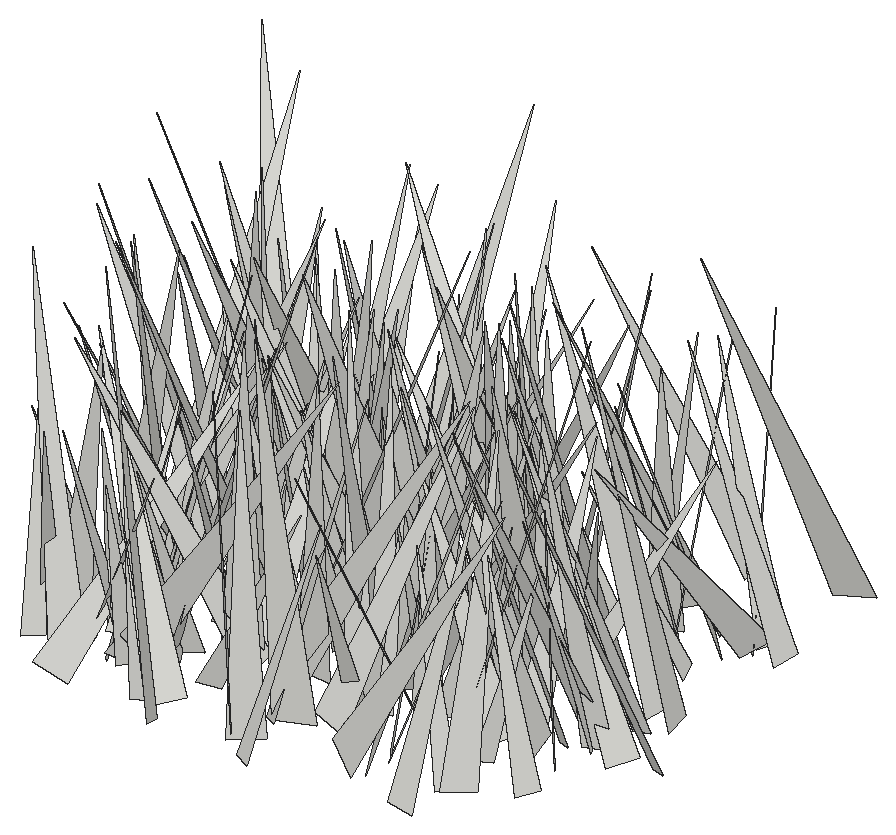
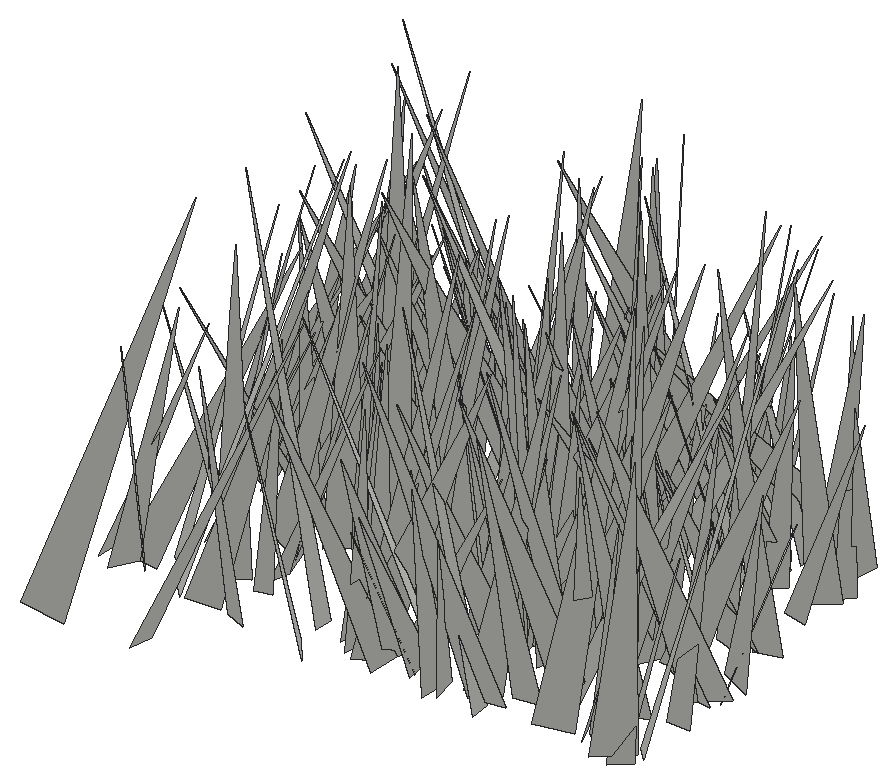
# SketchUp Ruby script. Lengths in inches.
U = 1.inch
M = Sketchup.active_model
def pt(a) = Geom::Point3d.new(a.map { |v| v * U })
def face(e, loops, mat)
  f = e.add_face(loops[0].map { |a| pt(a) })
  loops[1..].each { |l| e.add_face(l.map { |a| pt(a) }).erase! }
  f.material = f.back_material = mat if mat
  f
end
# faces: each face lists its corners as indices into pts; further lists are holes
def faces(e, pts, list, mat = nil) = list.each { |f| face(e, (f[0].is_a?(Array) ? f : [f]).map { |l| l.map { |i| pts[i] } }, mat) }
# xy, xz, yz: faces in a plane at the given z, y or x. An outline is a flat list of corners, or four numbers for a rectangle; further outlines are holes
def ring(l) = l.size == 4 ? [[l[0], l[1]], [l[2], l[1]], [l[2], l[3]], [l[0], l[3]]] : l.each_slice(2).to_a
def flat(e, list, mat, &to3) = list.each { |f| face(e, (f[0].is_a?(Array) ? f : [f]).map { |l| ring(l).map { |u, v| to3.(u, v) } }, mat) }
def xy(e, z, list, mat = nil) = flat(e, list, mat) { |x, y| [x, y, z] }
def xz(e, y, list, mat = nil) = flat(e, list, mat) { |x, z| [x, y, z] }
def yz(e, x, list, mat = nil) = flat(e, list, mat) { |y, z| [x, y, z] }
def lines(e, pts, list) = list.each { |a, b| e.add_line(pt(pts[a]), pt(pts[b])) }
# prism: a flat outline (further loops are holes) pulled along v
def prism(e, loops, v, mat = nil)
  f = face(e, loops, mat); d = Geom::Vector3d.new(v.map { |x| x * U })
  f.pushpull(f.normal.samedirection?(d) ? d.length : -d.length)
end
def box(e, o, s, mat = nil) = prism(e, [[o, [o[0] + s[0], o[1], o[2]], [o[0] + s[0], o[1] + s[1], o[2]], [o[0], o[1] + s[1], o[2]]]], [0, 0, s[2]], mat)
def at(x, y, z, deg = 0) = Geom::Transformation.translation(pt([x, y, z])) * Geom::Transformation.rotation(ORIGIN, Z_AXIS, deg.degrees)
def axes(o, x, y, z) = Geom::Transformation.new([*x, 0, *y, 0, *z, 0, *pt(o).to_a, 1])
def part(name) = M.definitions.add(name)
# library, detail: a bought-in or finely detailed component or shape, given as its bounding box
def library(name, o, s) = part(name).tap { |d| box(d.entities, o, s) }
def detail(e, o, s) = box(e.add_group.entities, o, s)
def put(e, d, t, mat = nil) = e.add_instance(d, t).tap { |i| i.material = mat if mat }
def group(e, t, mat = nil) = e.add_group.tap { |g| g.transformation = t; g.material = mat if mat }.entities
root = M.entities
c1 = part("fur_instance\#9")
p = [[0.8125,0,1.79],[0.67,-0.02,1.48],[0,-0.11,0],[0,0.11,0]]
faces(c1.entities,p,[[0,1,2,3]])
put(root,c1,axes([75.72,306.375,-27.1],[4.83002,3.67653,3.08875],[4.26917,-5.29337,-0.3752],[-2.19806,-2.20219,6.05848]))
put(root,c1,axes([76.89,305.76,-27.1],[3.45962,-4.50001,2.91683],[-5.02174,-3.93643,-0.1168],[-1.88153,2.2319,5.67498]))
put(root,c1,axes([77.69,304.53,-27.1],[2.30646,3.84948,0.31393],[3.83736,-2.32546,0.32205],[-0.43787,-0.10267,4.47599]))
put(root,c1,axes([80.25,306.78,-27.1],[3.77376,6.10396,1.49671],[5.76595,-2.66802,-3.65722],[2.50047,-3.05991,6.17449]))
put(root,c1,axes([72.33,305.65,-27.1],[-0.0394,4.36961,1.02441],[4.32756,-0.23455,1.1669],[-1.18959,-0.99797,4.2111]))
put(root,c1,axes([70.46,307.35,-27.1],[2.53184,-2.74895,1.13947],[-2.76231,-2.72751,-0.44237],[-1.1067,0.51894,3.71097]))
put(root,c1,axes([69.88,308.06,-27.1],[-4.44345,-1.97155,1.25823],[-1.71315,4.58269,1.13072],[1.59225,-0.57131,4.72787]))
put(root,c1,axes([73.58,304.73,-27.1],[-7.24108,-2.76695,1.69952],[-3.23599,6.49389,-3.21487],[0.2698,3.62643,7.05364]))
put(root,c1,axes([83.98,305.26,-27.1],[1.01663,5.56132,0.68679],[5.60282,-1.02017,-0.03274],[-0.09106,-0.68151,5.65338]))
put(root,c1,axes([68.67,307.44,-27.1],[4.5818,0.64032,0.1617],[0.65902,-4.5067,-0.82732],[-0.04299,-0.84188,4.55176]))
put(root,c1,axes([66.07,308.64,-27.1],[4.73789,-1.18845,0.72275],[-0.9672,-4.65874,-1.32025],[-0.99966,-1.12521,4.70287]))
put(root,c1,axes([77.43,307.71,-27.1],[-2.10134,6.53759,3.4605],[7.38552,2.05442,0.60354],[0.41142,-3.48856,6.84043]))
put(root,c1,axes([81.06,307.31,-27.1],[7.00496,3.81978,0.96353],[3.93839,-6.83549,-1.53416],[-0.09034,-1.80938,7.82984]))
put(root,c1,axes([73.15,306.09,-27.1],[-5.62336,3.63446,0.06059],[3.63174,5.6129,0.37548],[-0.15301,-0.3482,6.6851]))
put(root,c1,axes([78.87,309.48,-27.1],[0.77798,-4.23548,0.16889],[-4.23878,-0.77834,0.00619],[-0.02442,0.16723,4.30633]))
put(root,c1,axes([84.37,307.36,-27.1],[-3.97928,1.73175,0.54979],[1.73454,4.01483,-0.09183],[0.54094,-0.13447,4.3388]))
put(root,c1,axes([73.53,307.9,-27.1],[3.09859,-2.8989,0.71648],[-2.92503,-2.73871,1.56906],[0.60101,1.61681,3.94246]))
put(root,c1,axes([70.34,307.41,-27.1],[5.69226,-5.26322,0.96159],[-5.00885,-4.7486,3.65927],[1.88086,3.28288,6.8347]))
put(root,c1,axes([71.4,309.11,-27.1],[-5.49942,-3.45806,0.94275],[-3.51329,5.5426,-0.16378],[0.70973,0.64178,6.49422]))
put(root,c1,axes([74.0625,309.9375,-27.1],[-7.08449,-0.21202,0.14595],[-0.16992,6.87165,1.73429],[0.19334,-1.72965,6.8722]))
put(root,c1,axes([66.67,306.9,-27.1],[-4.24883,1.88722,0.42776],[1.75815,4.19597,-1.04876],[0.80838,0.79335,4.52927]))
put(root,c1,axes([80.23,310.84,-27.1],[-3.47678,-4.99975,0.07246],[-4.93171,3.44331,0.95532],[0.82523,-0.48669,6.01439]))
put(root,c1,axes([79.46,308.47,-27.1],[1.72384,-3.5656,0.8716],[-3.29525,-1.07913,2.10276],[1.61693,1.60212,3.35612]))
put(root,c1,axes([71.69,309.38,-27.1],[0.72019,-3.80208,0.86926],[-3.795,-0.88705,-0.73566],[-0.89965,0.69817,3.79912]))
put(root,c1,axes([68.43,309.53,-27.1],[3.6116,-2.54944,1.03868],[-2.46348,-3.75778,-0.65768],[-1.22872,0.0404,4.37159]))
put(root,c1,axes([68.17,306.91,-27.1],[-6.64184,2.29308,0.28161],[2.23011,6.58737,-1.04152],[0.60342,0.8944,6.94892]))
put(root,c1,axes([66.43,309.35,-27.1],[2.75053,-5.09352,1.52718],[-5.31748,-2.64324,0.76119],[-0.02665,1.70616,5.73847]))
put(root,c1,axes([86.78,308.78,-27.1],[-3.90024,1.94852,0.94584],[2.05782,3.9414,0.36592],[0.67579,-0.75618,4.3445]))
put(root,c1,axes([68.76,305.23,-27.1],[-3.50989,5.55769,0.51718],[4.45011,3.15505,-3.70364],[3.36927,1.62248,5.4305]))
put(root,c1,axes([73.36,309.95,-27.1],[4.72126,-4.87179,1.88096],[-5.03873,-4.91595,-0.08523],[-1.37242,1.28908,6.78361]))
put(root,c1,axes([75.08,309.59,-27.1],[4.55418,4.59674,3.34406],[5.23121,-5.06575,-0.16086],[-2.22422,-2.50228,6.46875]))
put(root,c1,axes([84.8,307.46,-27.1],[-5.4201,3.31702,1.28358],[3.06796,5.54385,-1.37151],[1.7994,0.53923,6.20476]))
put(root,c1,axes([69.67,307.125,-27.1],[3.36886,3.17868,0.5186],[2.75759,-3.23451,1.91201],[-1.66392,1.0752,4.2187]))
put(root,c1,axes([85.1,311.53,-27.1],[-7.14717,-1.7401,1.8273],[-1.33254,7.26397,1.70532],[2.14274,-1.28679,7.15555]))
put(root,c1,axes([75.9,310.64,-27.1],[0.59547,-6.22896,1.95156],[-6.50827,-0.41619,0.65745],[0.50087,1.99748,6.22272]))
put(root,c1,axes([66.56,310.77,-27.1],[-0.08918,-3.86635,0.81214],[-3.84672,-0.10019,-0.89937],[-0.90053,0.81086,3.76135]))
put(root,c1,axes([76.6875,307.3,-27.1],[3.68113,4.53912,0.36663],[4.24955,-3.59341,1.82137],[-1.63686,0.87892,5.5531]))
put(root,c1,axes([78.4375,308.35,-27.1],[1.11802,6.55656,0.88639],[6.4324,-0.86675,-1.70208],[1.54866,-1.13332,6.42972]))
put(root,c1,axes([81.57,307.78,-27.1],[4.34106,2.99141,0.28027],[2.79242,-4.19877,1.56351],[-1.10882,1.13738,5.03476]))
put(root,c1,axes([75.03,310.71,-27.1],[4.40787,6.56573,1.54887],[6.23945,-3.26461,-3.91775],[2.5646,-3.34225,6.86945]))
put(root,c1,axes([71.49,312.16,-27.1],[-3.69679,-5.87263,0.02895],[-5.78236,3.6339,-1.23044],[-1.02613,0.67962,6.82936]))
put(root,c1,axes([84.16,309.57,-27.1],[3.26385,-1.40609,1.47007],[-1.85279,-3.20219,1.05074],[-0.83985,1.59994,3.39496]))
put(root,c1,axes([83.07,309.98,-27.1],[4.24313,0.45781,1.20359],[0.34307,-4.39664,0.46288],[-1.24117,0.34981,4.24258]))
put(root,c1,axes([81.36,308.08,-27.1],[4.43621,4.25023,1.48293],[3.65379,-4.61591,2.29927],[-2.62932,0.75659,5.69717]))
put(root,c1,axes([69.42,310.12,-27.1],[6.44327,3.68852,1.42181],[3.82977,-6.4983,-0.49739],[-0.97955,-1.14429,7.40767]))
put(root,c1,axes([76.3,308.55,-27.1],[-6.09623,-2.24198,1.5344],[-2.70516,5.35755,-2.91953],[0.25098,3.28863,5.80232]))
put(root,c1,axes([68.91,308.79,-27.1],[-2.94733,3.27814,0.42411],[3.06608,2.92358,-1.29021],[1.23501,0.56503,4.21525]))
put(root,c1,axes([79.3,310.16,-27.1],[-0.34348,3.88251,1.09091],[4.02925,0.37671,-0.07204],[0.17064,-1.07988,3.89701]))
put(root,c1,axes([74.78,311.33,-27.1],[2.18952,-4.24382,2.13551],[-4.35668,-2.73133,-0.96101],[-1.89466,1.3763,4.67766]))
put(root,c1,axes([86.23,313.35,-27.1],[-1.07248,-7.00957,0.36815],[-6.96342,1.01561,-0.94825],[-0.88342,0.50425,7.02746]))
put(root,c1,axes([70.2,313.06,-27.1],[-1.799,-4.93024,0.4482],[-4.7112,1.85147,1.45641],[1.52075,-0.09654,5.04207]))
put(root,c1,axes([73.57,312.09,-27.1],[-3.74944,-6.99723,1.04952],[-6.92154,3.38084,-2.18706],[-1.468,1.93125,7.63127]))
put(root,c1,axes([86.12,311.03,-27.1],[3.3067,2.95122,2.18217],[3.23124,-3.73382,0.15332],[-1.74087,-1.32466,4.4295]))
put(root,c1,axes([83.76,311.19,-27.1],[-3.5373,3.73043,1.14853],[3.88761,3.22863,1.48666],[-0.34887,-1.84596,4.92122]))
put(root,c1,axes([82.12,312.63,-27.1],[3.81403,-1.87609,0.65313],[-1.66249,-3.78837,-1.17367],[-1.0874,-0.78844,4.08523]))
put(root,c1,axes([71.63,308.04,-27.1],[6.96857,3.90701,1.2479],[3.36407,-6.85211,2.66731],[-2.34628,1.77954,7.53068]))
put(root,c1,axes([76.64,313.21,-27.1],[6.75782,0.35235,2.65885],[1.16075,-6.88187,-2.03823],[-2.41791,-2.31896,6.45275]))
put(root,c1,axes([80.28,311.41,-27.1],[3.33409,-2.8819,1.80128],[-3.12207,-3.59416,0.02846],[-1.34262,1.20116,4.40689]))
put(root,c1,axes([72.57,312.99,-27.1],[2.27929,-4.31761,0.37807],[-4.29346,-2.30768,-0.46977],[-0.59235,0.11282,4.85966]))
put(root,c1,axes([79.76,312.16,-27.1],[-0.47471,-3.8388,0.84095],[-3.92781,0.49062,0.02236],[0.12592,0.83177,3.86797]))
put(root,c1,axes([83.41,308.91,-27.1],[6.6915,4.26773,1.20587],[3.94044,-6.72308,1.92792],[-2.03484,1.01512,7.69888]))
put(root,c1,axes([86.33,312.93,-27.1],[-4.22717,-2.44585,1.01456],[-2.28976,4.33627,0.91336],[1.32985,-0.3083,4.79759]))
put(root,c1,axes([67.24,313.69,-27.1],[-3.46246,-6.72611,1.90114],[-6.59046,3.84836,1.61233],[2.32826,0.89059,7.39118]))
put(root,c1,axes([75.32,312.98,-27.1],[3.88583,-1.17381,1.38743],[-0.79486,-4.04284,-1.19419],[-1.63432,-0.82466,3.87962]))
put(root,c1,axes([72.09,312.71,-27.1],[1.922,-3.18961,0.22781],[-3.1707,-1.86642,0.61867],[0.41494,0.51232,3.67219]))
put(root,c1,axes([68.85,311.06,-27.1],[3.76051,3.97563,0.83952],[4.01253,-3.81366,0.08642],[-0.64034,-0.54974,5.47171]))
put(root,c1,axes([89.28,312.75,-27.1],[-4.75874,-5.64309,0.42264],[-5.39038,4.3522,-2.58279],[-1.72245,1.97043,6.91515]))
put(root,c1,axes([85.59,312.22,-27.1],[-3.98273,-4.40716,0.90523],[-4.3967,3.55588,-2.0321],[-0.95477,2.0093,5.58174]))
put(root,c1,axes([75.32,313.49,-27.1],[3.57581,-3.48366,1.446],[-3.33217,-3.85124,-1.03819],[-1.76733,0.21279,4.88308]))
put(root,c1,axes([86.68,312.71,-27.1],[0.19192,-5.71021,2.24229],[-6.02696,-0.59408,-0.99702],[-1.14462,2.17066,5.62577]))
put(root,c1,axes([71.11,311.5,-27.1],[3.02903,2.92229,1.12241],[2.89072,-3.2105,0.55771],[-1.2014,-0.35704,4.17178]))
put(root,c1,axes([76.66,312.27,-27.1],[4.45392,4.12687,0.87812],[4.21021,-4.26347,-1.31776],[0.27618,-1.55927,5.92722]))
put(root,c1,axes([81.53,313.84,-27.1],[2.47243,-7.62212,2.09201],[-7.90302,-2.41845,0.52868],[-0.12434,2.1542,7.99563]))
put(root,c1,axes([65.71,313.32,-27.1],[-0.42435,-6.57592,2.54627],[-6.78158,1.0798,1.65847],[1.93298,2.34469,6.37748]))
put(root,c1,axes([82.26,315.08,-27.1],[5.27875,-5.42072,0.96709],[-5.29735,-5.36505,-1.15714],[-1.50251,-0.12916,7.47733]))
put(root,c1,axes([77.51,311.14,-27.1],[0.02975,6.47261,1.15989],[6.34372,-0.33363,1.69906],[-1.73125,-1.11127,6.2457]))
put(root,c1,axes([78.87,309.45,-27.1],[7.42059,-0.17453,3.00871],[-1.57677,-7.03899,3.48057],[-2.56838,3.81708,6.55601]))
put(root,c1,axes([78.27,311.49,-27.1],[-5.05186,2.37101,0.85511],[2.22237,5.09377,-0.9944],[1.18912,0.55319,5.49128]))
put(root,c1,axes([73.49,313.56,-27.1],[-2.97615,-4.05495,1.48787],[-4.26463,3.04523,-0.23114],[0.68511,1.34083,5.02461]))
put(root,c1,axes([79.25,312.14,-27.1],[6.564,-1.73993,0.0582],[-1.67851,-6.26496,2.01239],[0.46191,1.95953,6.48565]))
put(root,c1,axes([68.47,313.28,-27.1],[4.49917,3.28934,0.87918],[3.40387,-4.3112,-1.28935],[0.07989,-1.55853,5.42216]))
put(root,c1,axes([84.3,311.85,-27.1],[-1.65909,5.33475,1.21269],[5.33342,1.85943,-0.88312],[1.21852,-0.87506,5.51654]))
put(root,c1,axes([70.81,315.15,-27.1],[-0.56005,-4.94681,0.27227],[-4.82604,0.60667,1.09544],[1.12,0.14049,4.85639]))
put(root,c1,axes([71.62,313.03,-27.1],[0.44835,5.06558,1.88586],[5.29017,-0.02286,-1.19629],[1.10933,-1.93829,4.94267]))
put(root,c1,axes([73.21,311.27,-27.1],[-2.73527,5.15415,0.70761],[4.98067,2.82527,-1.3261],[1.50298,0.0175,5.68229]))
put(root,c1,axes([87.96,312.47,-27.1],[-2.08516,6.03207,0.25096],[5.29839,1.7011,3.1353],[-2.89412,-1.23172,5.5591]))
put(root,c1,axes([86.47,314.58,-27.1],[-6.23663,-1.3966,0.55844],[-1.37103,6.25805,0.33911],[0.61857,-0.21031,6.38209]))
put(root,c1,axes([76.94,313.36,-27.1],[6.19791,-1.23637,0.25272],[-1.26158,-6.10069,1.0939],[-0.02993,1.12232,6.22464]))
put(root,c1,axes([75.44,315.5,-27.1],[1.50286,-5.49819,1.33251],[-5.18917,-1.88889,-1.94134],[-2.25347,0.68284,5.35909]))
put(root,c1,axes([81.19,311.29,-27.1],[-4.89219,1.92037,1.37183],[1.09822,4.64707,-2.5888],[2.08893,2.05431,4.57377]))
put(root,c1,axes([87.12,314.57,-27.1],[-0.99125,-4.30354,0.98962],[-4.28593,0.69339,-1.27766],[-1.06332,1.21702,4.22737]))
put(root,c1,axes([78.98,315.125,-27.1],[-6.42976,0.15301,2.02637],[0.5172,6.6259,1.14077],[1.96522,-1.24316,6.3296]))
put(root,c1,axes([67.26,316.42,-27.1],[-6.10704,-5.17922,1.29191],[-4.99805,6.23748,1.37932],[1.87424,-0.24245,7.88782]))
put(root,c1,axes([66.34,313.33,-27.1],[3.26284,4.45559,0.15103],[4.26787,-3.06768,-1.7017],[1.28856,-1.1217,5.25381]))
put(root,c1,axes([74.08,312.47,-27.1],[7.5502,3.19495,0.69372],[3.12341,-7.56468,0.84526],[-0.96605,0.51231,8.15468]))
put(root,c1,axes([83.39,316.02,-27.1],[5.22724,-1.35677,0.09683],[-1.28473,-5.05093,-1.4184],[-0.44684,-1.34966,5.21086]))
put(root,c1,axes([74.56,315.53,-27.1],[-6.62778,2.24684,1.33683],[2.5489,6.36376,1.94128],[0.58185,-2.2841,6.72363]))
put(root,c1,axes([77.29,314.9,-27.1],[2.95876,-6.29379,1.88961],[-6.54545,-2.63888,1.45948],[0.58268,2.31543,6.79971]))
put(root,c1,axes([77.6,317.09,-27.1],[6.21031,-0.46369,2.15458],[0.49806,-5.98034,-2.72263],[-2.14689,-2.7287,5.60092]))
put(root,c1,axes([84.37,315.41,-27.1],[-1.75901,-5.06572,0.78099],[-4.97011,1.48393,-1.5689],[-1.25276,1.22556,5.12778]))
put(root,c1,axes([69.07,313.95,-27.1],[3.47844,1.93474,0.04271],[1.93521,-3.47755,-0.07868],[0.00093,-0.08952,3.97952]))
put(root,c1,axes([71.29,311.52,-27.1],[-5.44791,2.04028,1.98238],[0.64646,5.0587,-3.42987],[2.77031,2.83181,4.69878]))
put(root,c1,axes([68.04,312.43,-27.1],[-4.70225,1.57903,0.9136],[0.9953,4.33742,-2.37389],[1.52885,2.03289,4.35536]))
put(root,c1,axes([73.96,318.25,-27.1],[5.79186,-5.56058,1.06137],[-5.14067,-5.80215,-2.34538],[-2.37068,-1.00358,7.67886]))
put(root,c1,axes([68.65,316.39,-27.1],[7.59105,-2.36712,2.02897],[-2.18853,-7.84946,-0.96967],[-2.22043,-0.35586,7.89221]))
put(root,c1,axes([72.45,316.44,-27.1],[5.8288,-3.89293,1.62458],[-3.86791,-6.0381,-0.59132],[-1.68328,0.3943,6.98428]))
put(root,c1,axes([71.9,313.29,-27.1],[2.76553,6.92914,2.18566],[6.51494,-3.40021,2.53621],[-3.21647,-0.92942,7.01632]))
put(root,c1,axes([67.41,316.06,-27.1],[-3.27496,5.22829,1.96451],[5.47571,2.5569,2.32348],[-1.10043,-2.83671,5.71505]))
put(root,c1,axes([70.7,318.28,-27.1],[0.98136,-7.62341,0.77855],[-7.49654,-1.11781,-1.49599],[-1.58884,0.56543,7.53933]))
put(root,c1,axes([78.21,318.34,-27.1],[0.34985,-8.1007,0.677],[-7.9597,-0.20383,1.67442],[1.6501,0.73429,7.93347]))
put(root,c1,axes([73.08,315.99,-27.1],[-8.06314,0.9505,0.88883],[1.02226,8.07835,0.63476],[0.80526,-0.7379,8.09412]))
put(root,c1,axes([87.72,315.75,-27.1],[-7.02647,-2.17808,1.10616],[-2.29777,7.03636,-0.74079],[0.82938,1.04138,7.31892]))
put(root,c1,axes([64.94,316.76,-27.1],[-3.14416,-1.79317,0.28571],[-1.75542,3.14785,0.43854],[0.46429,-0.24163,3.59289]))
put(root,c1,axes([81.59,316.53,-27.1],[4.24659,-4.94069,2.32668],[-5.22174,-4.53655,-0.10277],[-1.59916,1.69313,6.51409]))
put(root,c1,axes([73.99,314.34,-27.1],[-6.21207,0.31771,0.7174],[0.09871,5.99609,-1.80072],[0.77837,1.77522,5.95384]))
put(root,c1,axes([81.63,314.85,-27.1],[-5.20455,-0.25594,1.25726],[-0.61037,5.11409,-1.48563],[1.12857,1.58561,4.99457]))
put(root,c1,axes([83.66,317.59,-27.1],[-3.27464,-6.78559,1.40651],[-6.92909,3.22889,-0.5548],[0.10135,1.50857,7.51397]))
put(root,c1,axes([74.65,317.38,-27.1],[2.8154,-3.04723,0.70248],[-2.99803,-2.89898,-0.55973],[-0.88933,0.126,4.11081]))
put(root,c1,axes([86.71,316.27,-27.1],[-8.26176,0.40654,0.83522],[0.41692,8.30295,0.08258],[0.83009,-0.12394,8.27135]))
put(root,c1,axes([72.48,317.15,-27.1],[6.13982,-1.63324,0.91897],[-1.58888,-6.20592,-0.4139],[-0.99371,-0.16841,6.33984]))
put(root,c1,axes([67.33,316.4,-27.1],[2.36922,2.94645,1.17355],[3.15581,-2.33594,-0.5062],[-0.31572,-1.23846,3.7468]))
put(root,c1,axes([67.6,315.74,-27.1],[2.29816,3.3477,0.63042],[3.39972,-2.30202,-0.16916],[-0.21536,-0.61617,4.05709]))
put(root,c1,axes([72.42,317.84,-27.1],[-0.76172,-5.93829,1.58025],[-5.83151,1.20063,1.7008],[1.93753,1.27903,5.74028]))
put(root,c1,axes([72.01,317.21,-27.1],[0.25447,-5.59234,1.88155],[-5.79418,0.11887,1.13692],[1.11444,1.89496,5.48146]))
put(root,c1,axes([65.3125,315.6,-27.1],[0.45308,4.94253,1.25959],[4.74966,-0.86975,1.70432],[-1.859,-1.01755,4.66145]))
put(root,c1,axes([81.02,316.73,-27.1],[3.81307,5.29138,3.34018],[5.75803,-4.49829,0.55278],[-2.44962,-2.33704,6.49867]))
put(root,c1,axes([68.27,318.67,-27.1],[-3.1759,-6.57357,0.78945],[-6.61199,3.10387,-0.75436],[-0.34161,1.03711,7.26148]))
put(root,c1,axes([69.45,315.82,-27.1],[-1.35626,4.67986,0.4324],[4.48876,1.15652,1.56235],[-1.3925,-0.82998,4.61514]))
put(root,c1,axes([82.23,318.41,-27.1],[-5.80555,-2.80529,1.19859],[-2.69051,5.92298,0.83076],[1.43785,-0.24369,6.39405]))
put(root,c1,axes([83.24,315.77,-27.1],[2.06268,4.77096,0.10661],[4.57909,-1.94603,-1.50762],[1.34363,-0.69206,4.97431]))
put(root,c1,axes([72.28,318.12,-27.1],[-3.33376,-1.76985,1.3611],[-1.54667,3.5947,0.88593],[1.61021,-0.21143,3.66899]))
put(root,c1,axes([71.61,316.14,-27.1],[0.20171,6.63601,2.13173],[6.14884,-1.17367,3.07178],[-3.28217,-1.79094,5.8857]))
put(root,c1,axes([64.98,319.11,-27.1],[-0.80762,-5.18,0.70533],[-5.16495,0.90095,0.70267],[0.80822,0.5814,5.19528]))
put(root,c1,axes([85.72,318.81,-27.1],[-4.15133,-1.53142,0.10873],[-1.49707,4.10736,0.69206],[0.34034,-0.61232,4.37033]))
put(root,c1,axes([74.31,317.88,-27.1],[3.95435,2.54343,1.52337],[2.80761,-4.0284,-0.56212],[-0.95239,-1.31514,4.66797]))
put(root,c1,axes([68.22,321.91,-27.1],[7.18044,-3.7228,0.21814],[-3.29243,-6.55088,-3.42221],[-1.75122,-2.94828,7.32847]))
put(root,c1,axes([86.55,321.57,-27.1],[3.78174,-4.82109,0.17581],[-4.12071,-3.34423,-3.06777],[-2.50869,-1.77444,5.30408]))
put(root,c1,axes([71.15,318.23,-27.1],[5.93404,-1.49093,1.99542],[-1.59561,-6.23409,0.08712],[-1.91274,0.57506,6.11785]))
put(root,c1,axes([85.39,320.89,-27.1],[-4.26482,-5.03014,0.77761],[-4.82923,4.31941,1.45497],[1.60794,-0.36894,6.43227]))
put(root,c1,axes([65.44,317.375,-27.1],[2.30365,5.6713,0.71156],[5.64313,-2.13475,-1.25489],[0.90837,-1.12069,5.9913]))
put(root,c1,axes([83.89,320.55,-27.1],[-3.75985,-4.2409,1.14983],[-3.97997,3.92819,1.47409],[1.86202,-0.16705,5.47255]))
put(root,c1,axes([82.05,319.53,-27.1],[-5.02334,-0.16728,0.55191],[-0.071,4.98153,0.86367],[0.57231,-0.85028,4.95137]))
put(root,c1,axes([69.41,319.11,-27.1],[-5.59942,-5.49473,0.70955],[-5.42162,5.22657,-2.3104],[-1.14084,2.13071,7.49717]))
put(root,c1,axes([78,319.07,-27.1],[-6.68615,-0.01766,0.93467],[0.01232,6.74773,0.2156],[0.93476,-0.21523,6.6827]))
put(root,c1,axes([64.89,322.39,-27.1],[-1.50636,-7.45489,0.25307],[-6.77182,1.47502,3.14252],[3.12761,-0.39686,6.92598]))
put(root,c1,axes([84.23,322.37,-27.1],[-5.99255,-5.60768,0.41861],[-5.37957,5.89507,1.95969],[1.63755,-1.155,7.96972]))
put(root,c1,axes([76.13,322.13,-27.1],[6.61822,-2.56323,1.80089],[-1.74555,-6.51281,-2.85492],[-2.60123,-2.15113,6.49773]))
put(root,c1,axes([81.86,320.6875,-27.1],[-0.45629,-4.37673,0.42276],[-4.25435,0.54685,1.06962],[1.11127,0.29645,4.26847]))
put(root,c1,axes([72.79,319.4,-27.1],[-3.17,-4.98135,1.74667],[-5.27871,2.99065,-1.05117],[-0.00204,2.03858,5.81015]))
put(root,c1,axes([72.33,320.62,-27.1],[-2.39227,-3.29447,0.41561],[-3.24315,2.42809,0.57931],[0.71291,-0.00928,4.03]))
put(root,c1,axes([72.91,318.75,-27.1],[4.25693,-2.37845,0.80532],[-2.50825,-3.95225,1.586],[0.11926,1.77474,4.61119]))
put(root,c1,axes([83.29,320.61,-27.1],[3.25628,-4.96201,1.27437],[-5.08219,-3.31911,0.06246],[-0.64574,1.10043,5.93473]))
put(root,c1,axes([69.7,318.33,-27.1],[-4.60941,2.24833,0.68921],[2.12734,4.63308,-0.88638],[1.00221,0.50623,5.05134]))
put(root,c1,axes([78.83,321.2,-27.1],[7.66511,2.45698,1.17946],[2.70747,-7.26796,-2.45522],[-0.3122,-2.70587,7.66567]))
put(root,c1,axes([77.63,321.46,-27.1],[-4.01189,-2.17426,1.82805],[-1.57492,4.33524,1.69992],[2.36407,-0.80168,4.23473]))
put(root,c1,axes([71.61,321.47,-27.1],[3.35042,-5.0359,1.55374],[-4.92978,-3.64566,-1.18576],[-1.86322,0.59037,5.93123]))
put(root,c1,axes([76.94,320.62,-27.1],[0.54293,-5.17192,1.62827],[-5.42158,-0.49338,0.24063],[0.08095,1.64396,5.19477]))
put(root,c1,axes([70.75,317.8,-27.1],[0.90222,6.95991,0.72818],[6.98982,-0.93156,0.24337],[-0.33621,-0.69025,7.01392]))
put(root,c1,axes([66.5,319.57,-27.1],[-0.43128,5.47544,2.09207],[5.72554,0.84273,-1.02531],[1.25517,-1.9628,5.39585]))
put(root,c1,axes([64.72,321.39,-27.1],[-3.11694,-3.18155,0.61605],[-3.14817,3.17551,0.47138],[0.76862,0.10457,4.42892]))
put(root,c1,axes([82.99,322.56,-27.1],[2.63198,-5.20128,0.6124],[-4.94839,-2.69423,-1.6156],[-1.71515,-0.20845,5.60093]))
put(root,c1,axes([65.25,317.16,-27.1],[-3.2389,7.2108,0.31573],[7.08918,3.2432,-1.34571],[1.35602,0.26802,7.78942]))
put(root,c1,axes([75.41,320.6,-27.1],[-3.7614,2.09395,0.36046],[2.10674,3.58022,1.1859],[-0.27609,-1.20834,4.13841]))
put(root,c1,axes([65.89,320.55,-27.1],[-2.9488,-2.48385,0.84804],[-2.61567,2.88641,-0.64107],[0.2167,1.04076,3.80183]))
put(root,c1,axes([85.24,318.37,-27.1],[4.44395,3.96646,1.43413],[3.47391,-4.62357,2.02305],[-2.39195,0.65422,5.60257]))
put(root,c1,axes([67.03,321.69,-27.1],[-3.51503,-1.89548,0.64915],[-1.82323,3.56963,0.55065],[0.83071,-0.18586,3.95538]))
put(root,c1,axes([69.58,319.33,-27.1],[-0.94911,6.39885,1.08787],[6.32075,1.1611,-1.31509],[1.4754,-0.85797,6.33377]))
put(root,c1,axes([73.15,321.61,-27.1],[5.8637,3.4963,0.04079],[3.31459,-5.53283,-2.23832],[1.11324,-1.94227,6.44958]))
put(root,c1,axes([77.11,320.56,-27.1],[-5.54363,5.04114,0.10568],[4.92423,5.3789,1.72499],[-1.08457,-1.34553,7.29173]))
put(root,c1,axes([70.92,322.54,-27.1],[6.83601,2.20523,1.02382],[2.40175,-6.59991,-1.82073],[-0.37792,-2.05437,6.94831]))
put(root,c1,axes([66.55,321.72,-27.1],[-2.19445,-3.56039,1.55722],[-3.85398,2.22319,-0.34801],[0.4981,1.5159,4.16783]))
put(root,c1,axes([87.85,321.54,-27.1],[-5.92651,0.06077,0.05927],[0.05827,5.92175,-0.24529],[0.06173,0.24468,5.92174]))
put(root,c1,axes([70.07,321.01,-27.1],[-0.06431,5.36711,1.48252],[5.54585,0.19413,-0.46222],[0.49719,-1.47116,5.34755]))
put(root,c1,axes([76.99,321.63,-27.1],[-4.7956,1.01448,1.55419],[0.95492,5.04106,-0.34401],[1.59148,0.0322,4.88965]))
put(root,c1,axes([86.79,322.15,-27.1],[-5.29366,2.0126,1.17564],[2.12712,5.36423,0.39489],[0.95291,-0.79376,5.64955]))
put(root,c1,axes([75.52,322.03,-27.1],[5.25696,-1.00652,0.21452],[-1.02902,-5.15697,1.02054],[-0.01477,1.04274,5.25426]))
put(root,c1,axes([81.4,322.78,-27.1],[1.95636,4.4496,1.57567],[4.70552,-1.97342,-0.26957],[-0.3738,-1.55425,4.8532]))
put(root,c1,axes([72.83,322.1,-27.1],[-3.84179,0.25674,0.88435],[-0.00822,3.78425,-1.13434],[0.92083,1.10494,3.67947]))
put(root,c1,axes([86.67,321.18,-27.1],[3.82585,4.29132,1.89582],[3.55577,-4.24822,2.44044],[-3.06039,0.42878,5.20545]))
put(root,c1,axes([74.38,321.46,-27.1],[-4.08665,1.67614,0.95166],[1.15635,3.91687,-1.93308],[1.54207,1.50482,3.97156]))
put(root,c1,axes([74.78,321.5,-27.1],[2.09645,3.63188,0.13416],[3.39461,-2.01213,1.42535],[-1.29816,0.60366,3.94386]))
put(root,c1,axes([73.05,322.29,-27.1],[-4.76791,1.69378,1.39092],[1.4281,4.92716,-1.10462],[1.66255,0.62512,4.93778]))
put(root,c1,axes([65.43,322.08,-27.1],[-5.44191,5.3364,0.6963],[5.36336,5.45938,0.07682],[0.44311,-0.54257,7.6214]))
put(root,c1,axes([86.87,326.5,-27.1],[0.82289,-7.98079,0.80674],[-7.83354,-0.97405,-1.64552],[-1.72608,0.61581,7.85254]))
put(root,c1,axes([75.4375,321.06,-27.1],[-4.827,3.94667,0.05385],[3.76525,4.62978,-1.80751],[1.18405,1.36675,5.96733]))
put(root,c1,axes([71.1,321.91,-27.1],[0.33819,7.69063,1.05021],[7.70297,-0.20312,-0.99305],[0.95553,-1.08446,7.63374]))
put(root,c1,axes([78.3125,323.02,-27.1],[3.87453,3.49507,1.24049],[3.40824,-4.0629,0.80191],[-1.46226,-0.20898,5.15601]))
put(root,c1,axes([82.93,326.03,-27.1],[-6.88482,-1.0416,0.48285],[-0.90858,6.73783,1.57954],[0.70182,-1.49517,6.78165]))
